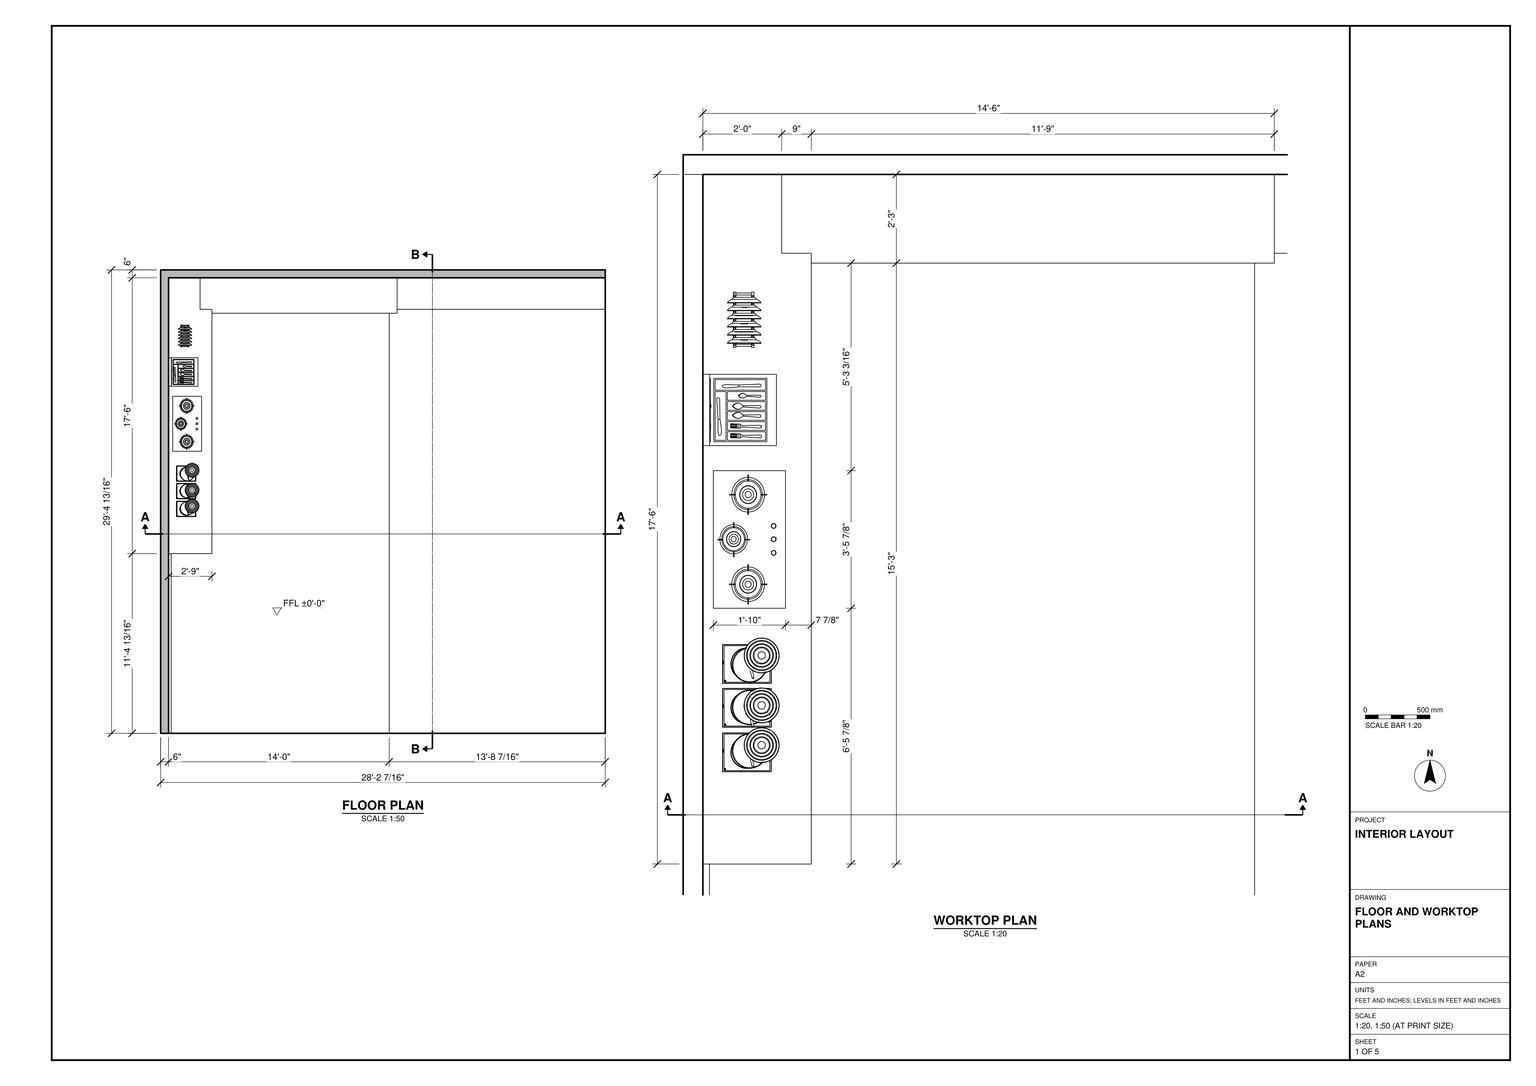
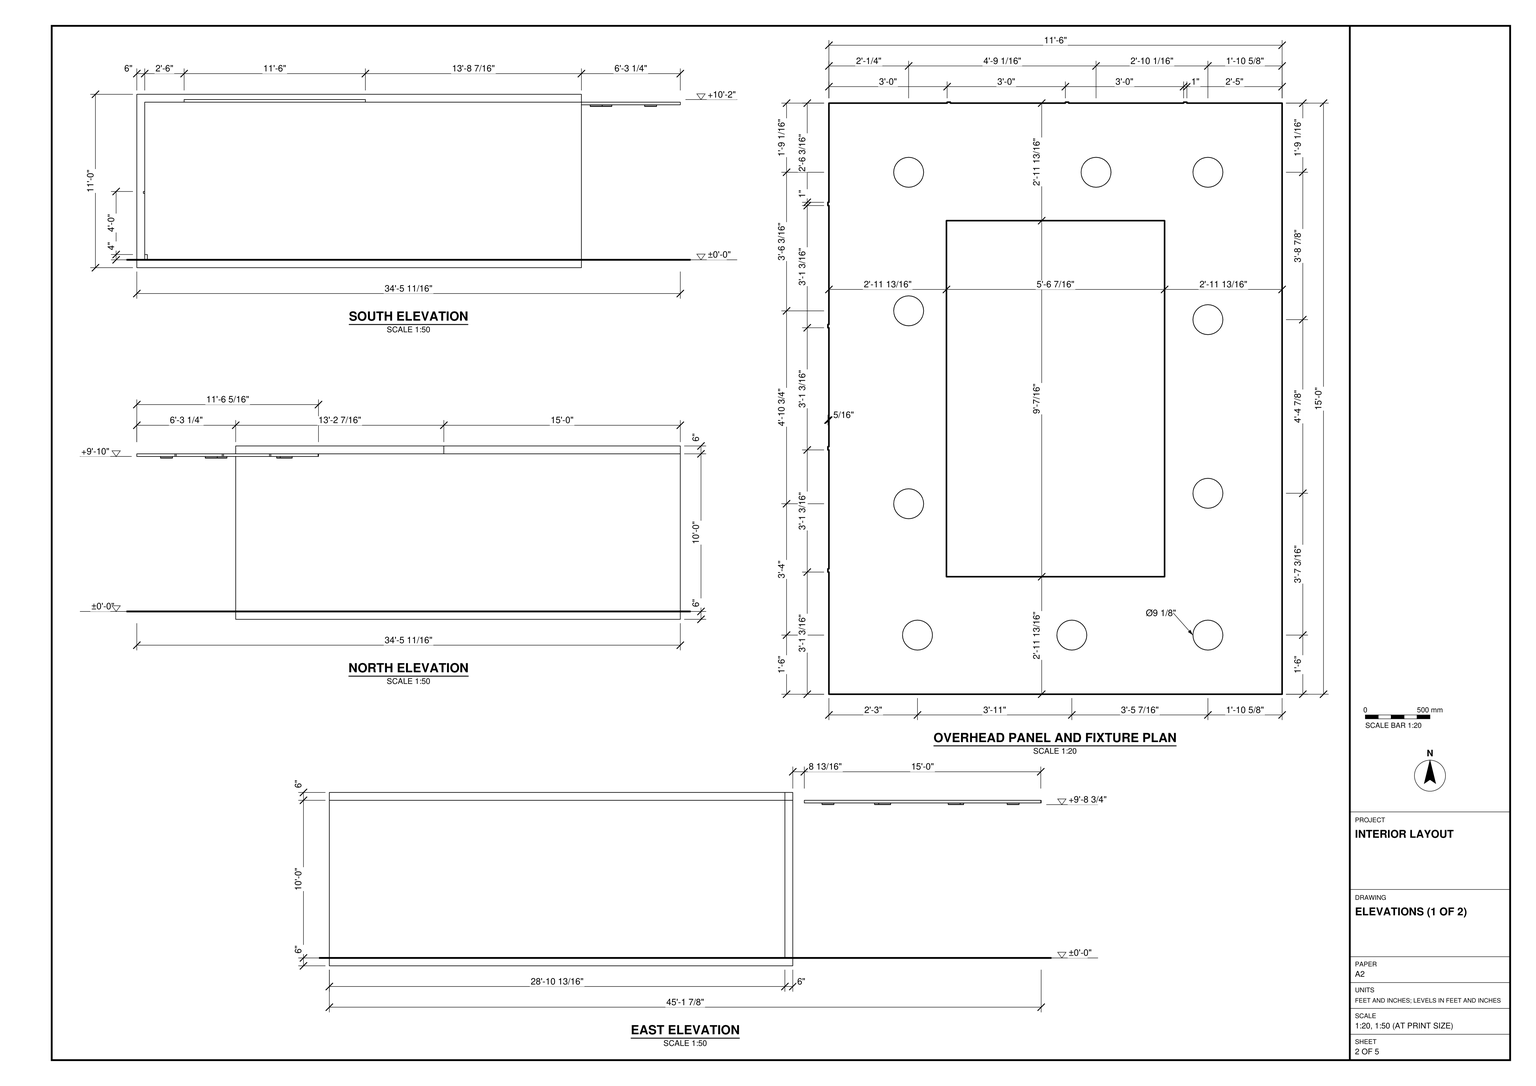
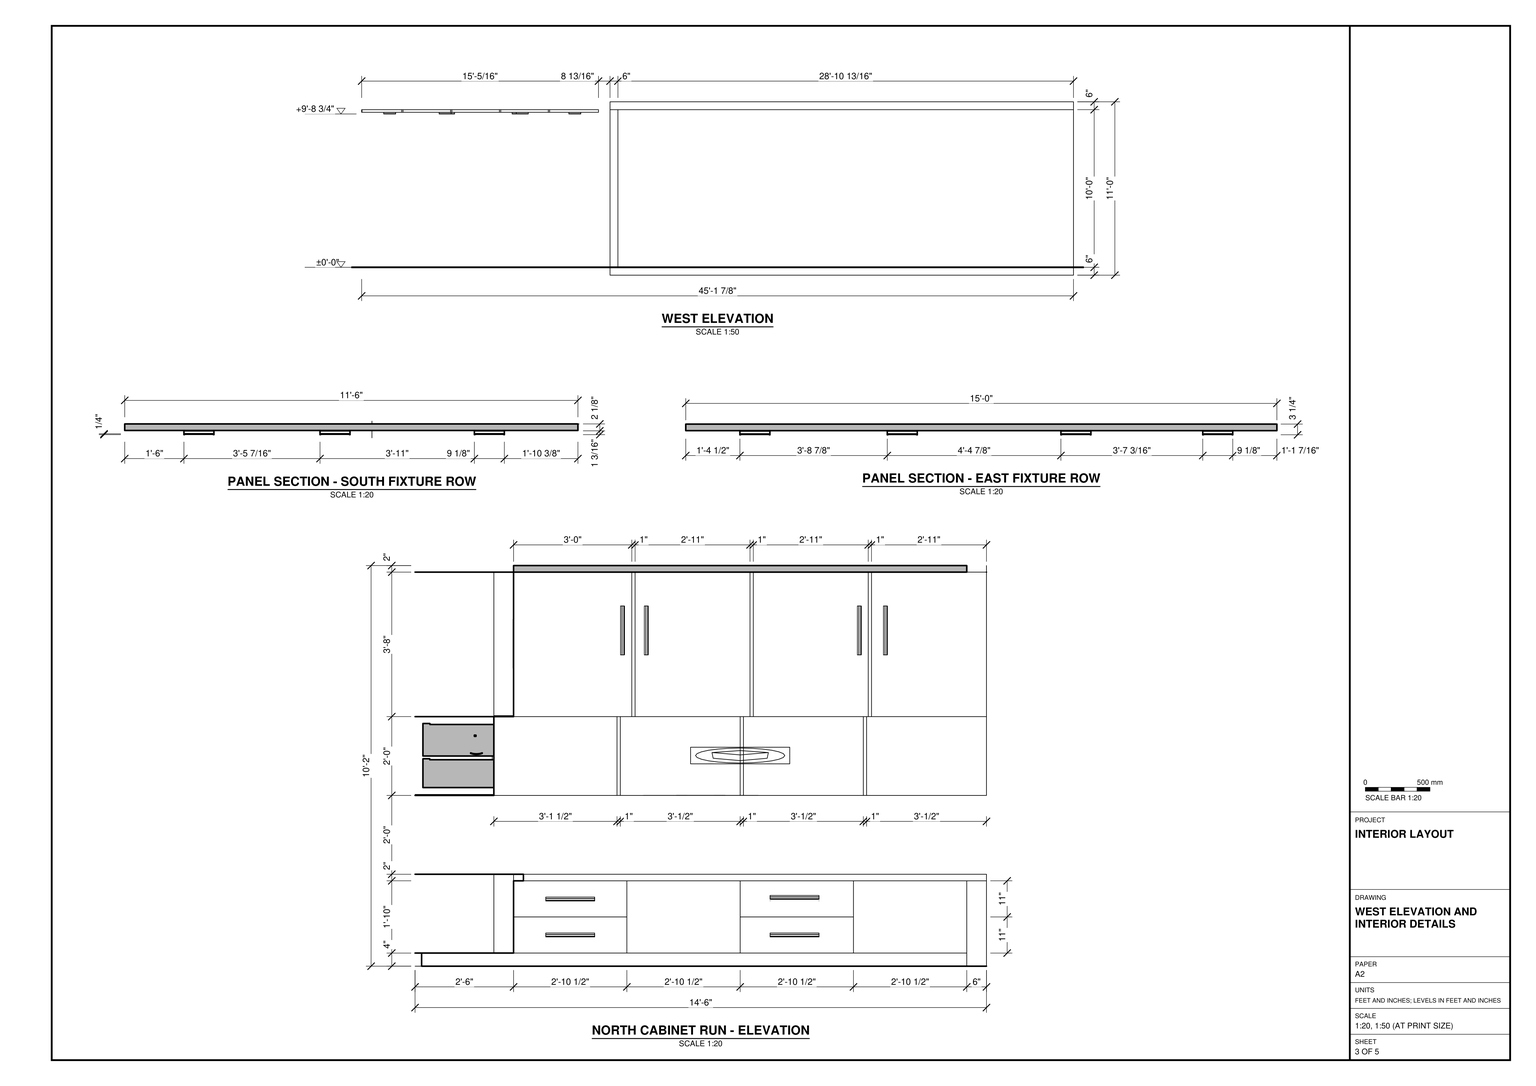
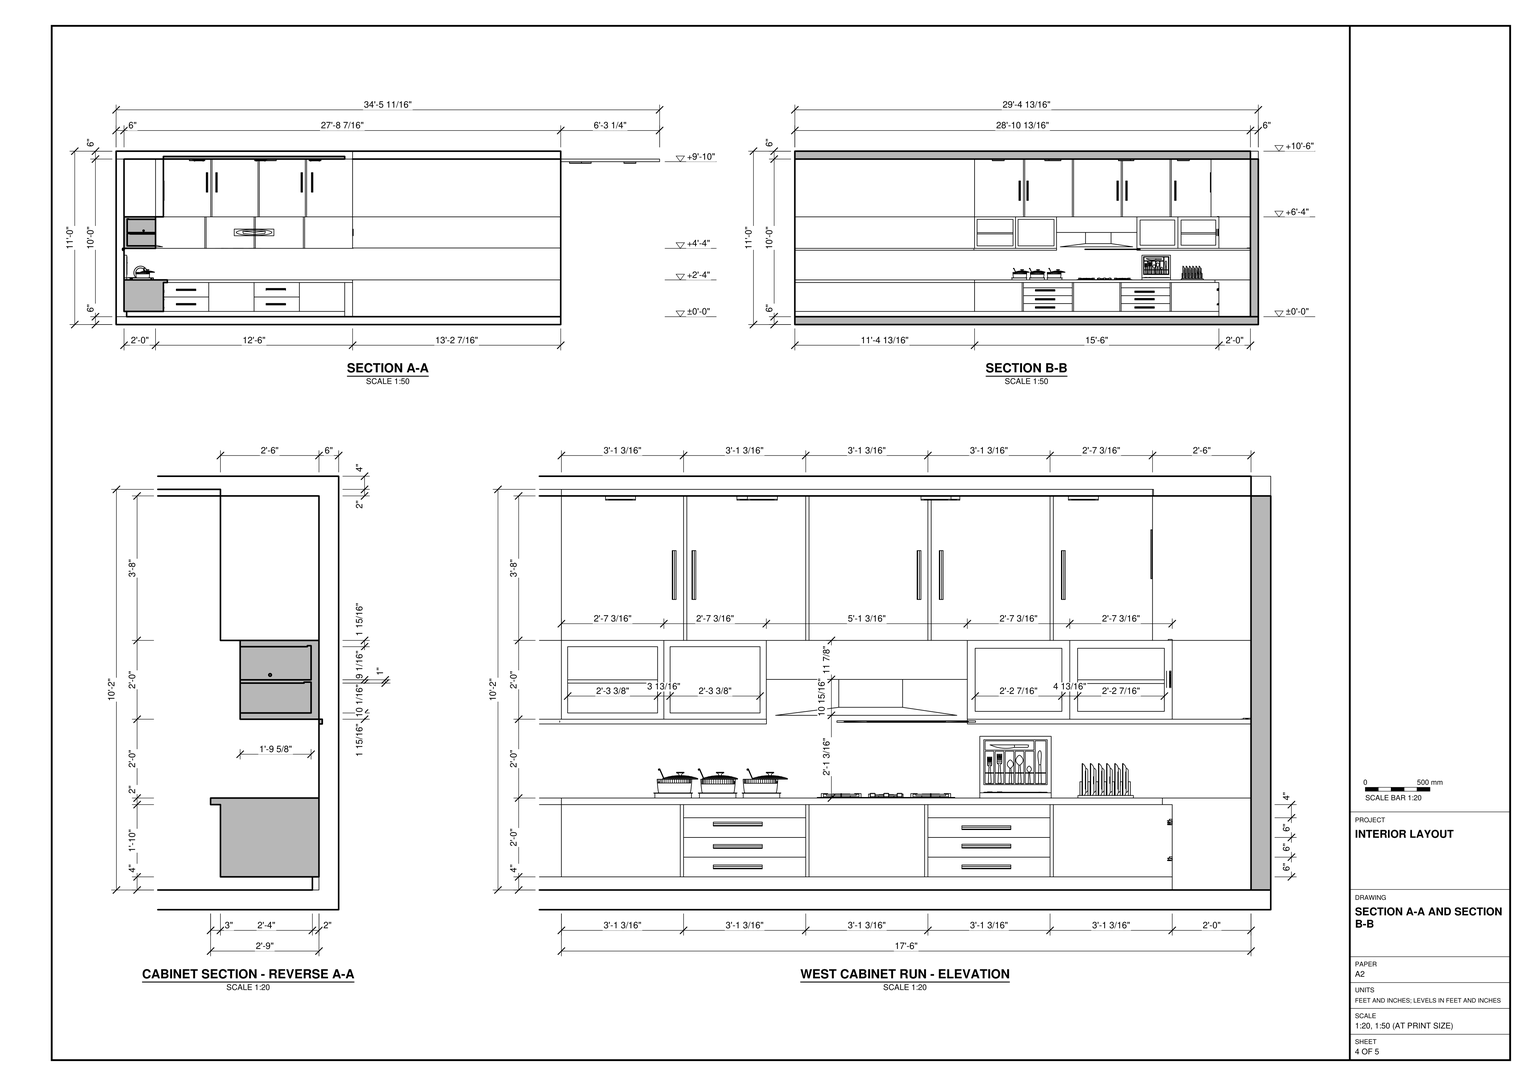
Build the kitchen interior in SketchUp from task_files/diagram_01.pdf. Work in feet and inches. The complete model, including the separate overhead panel, measures 34'-5 11/16" along X, 45'-1 7/8" along Y and 11'-0" along Z. Set the finished floor at ±0'-0". Use the floor plan for the room footprint rather than treating the overall model extents as wall lengths.

Model the floor slab, the adjoining north and west walls, and the slab above the room. Follow the 6" shell thicknesses and the 10'-0" clear height shown in the plans and elevations. Fit the worktop along the west wall and turn it along the north wall, leaving the main floor area open. Match the stepped outline at the corner. Use the north cabinet elevation to set out the plinth, alternating drawer stacks and plain base fronts, the clear space above the worktop, and the two tiers of wall cabinetry. Place the cooktop, utensil tray and cookware in their indicated positions on the west run.

Model the separate overhead panel at the offset shown in the elevations, with its central rectangular field and the fixtures arranged around it. Decor and loose items may be any suitable library components. Keep the shell elements and each furniture or joinery piece in separate groups or components, and use components for repeated parts. Save one SketchUp model as output_files/kitchen_with_l_shaped_joinery_and_overhead_panel.skp.

# SketchUp Ruby script. Lengths in inches.
U = 1.inch
M = Sketchup.active_model
def pt(a) = Geom::Point3d.new(a.map { |v| v * U })
def face(e, loops, mat)
  f = e.add_face(loops[0].map { |a| pt(a) })
  loops[1..].each { |l| e.add_face(l.map { |a| pt(a) }).erase! }
  f.material = f.back_material = mat if mat
  f
end
# faces: each face lists its corners as indices into pts; further lists are holes
def faces(e, pts, list, mat = nil) = list.each { |f| face(e, (f[0].is_a?(Array) ? f : [f]).map { |l| l.map { |i| pts[i] } }, mat) }
# xy, xz, yz: faces in a plane at the given z, y or x. An outline is a flat list of corners, or four numbers for a rectangle; further outlines are holes
def ring(l) = l.size == 4 ? [[l[0], l[1]], [l[2], l[1]], [l[2], l[3]], [l[0], l[3]]] : l.each_slice(2).to_a
def flat(e, list, mat, &to3) = list.each { |f| face(e, (f[0].is_a?(Array) ? f : [f]).map { |l| ring(l).map { |u, v| to3.(u, v) } }, mat) }
def xy(e, z, list, mat = nil) = flat(e, list, mat) { |x, y| [x, y, z] }
def xz(e, y, list, mat = nil) = flat(e, list, mat) { |x, z| [x, y, z] }
def yz(e, x, list, mat = nil) = flat(e, list, mat) { |y, z| [x, y, z] }
def lines(e, pts, list) = list.each { |a, b| e.add_line(pt(pts[a]), pt(pts[b])) }
# prism: a flat outline (further loops are holes) pulled along v
def prism(e, loops, v, mat = nil)
  f = face(e, loops, mat); d = Geom::Vector3d.new(v.map { |x| x * U })
  f.pushpull(f.normal.samedirection?(d) ? d.length : -d.length)
end
def box(e, o, s, mat = nil) = prism(e, [[o, [o[0] + s[0], o[1], o[2]], [o[0] + s[0], o[1] + s[1], o[2]], [o[0], o[1] + s[1], o[2]]]], [0, 0, s[2]], mat)
def at(x, y, z, deg = 0) = Geom::Transformation.translation(pt([x, y, z])) * Geom::Transformation.rotation(ORIGIN, Z_AXIS, deg.degrees)
def axes(o, x, y, z) = Geom::Transformation.new([*x, 0, *y, 0, *z, 0, *pt(o).to_a, 1])
def part(name) = M.definitions.add(name)
# library, detail: a bought-in or finely detailed component or shape, given as its bounding box
def library(name, o, s) = part(name).tap { |d| box(d.entities, o, s) }
def detail(e, o, s) = box(e.add_group.entities, o, s)
def put(e, d, t, mat = nil) = e.add_instance(d, t).tap { |i| i.material = mat if mat }
def group(e, t, mat = nil) = e.add_group.tap { |g| g.transformation = t; g.material = mat if mat }.entities
root = M.entities
M.materials.add("Color_0").color = [255, 255, 255]
M.materials.add("DefaultMaterial32").color = [145, 100, 66]
M.materials.add("Generic").color = [223, 223, 223]
M.materials.add("Teddy_Shoes").color = [231, 232, 232]
M.materials.add("[Carrera Marble]").color = [207, 207, 207]
M.materials.add("[Carrera Marble]2").color = [207, 207, 207]
M.materials.add("[Carrera Marble]3").color = [207, 207, 207]
M.materials.add("[Color_003]").color = [232, 232, 232]
M.materials.add("[Translucent Glass Gray]").color = [128, 128, 128]
M.materials["[Translucent Glass Gray]"].alpha = 0.5
M.materials.add("[_0060_GrassGreen_]").color = [200, 200, 200]
c1 = library("Bosch Stove",[0,0,0],[36.22,20.12,1.38])
c2 = library("PLATE",[-1.81,0,33.86],[10.25,10.83,10.53])
c3 = library("bottle",[0,0,0],[211.8125,112.55,469.29])
c4 = library("top",[0,0,0],[118.11,118.11,64.96])
c5 = library("pump",[0,0,-431.92],[75.04,51.18,479.16])
c6 = library("cap",[0,0,0],[90.55,90.55,133.86])
c7 = library("Group\#3",[0,0,0],[19.58,60.1,12.07])
c8 = part("E")
xy(c8.entities,0.2,[[6.05,0,4.93,0.4,4.54,0.95,4.41,1.79,4.41,31.375,4.54,32.22,4.93,32.77,6.05,33.17,21.79,33.17,22.16,33.06,22.43,32.73,22.59,32.15,22.66,31.3,22.59,30.49,22.43,29.92,22.16,29.6,21.79,29.5,8.82,29.5,8.82,19.1,19.94,19.1,20.3125,18.98,20.59,18.66,20.76,18.1,20.8125,17.25,20.76,16.46,20.59,15.92,20.3125,15.62,19.94,15.53,8.82,15.53,8.82,3.67,21.97,3.67,22.34,3.5625,22.63,3.24,22.8125,2.68,22.86,1.82,22.8125,1.01,22.63,0.4375,22.34,0.1,21.97,0]])
c9 = part("S")
xy(c9.entities,0.2,[[10.94,0,7.86,0.28,5.32,0.97,3.45,1.82,2.4,2.5625,1.96,3.34,1.82,4.61,1.87,5.55,2.02,6.15,2.28,6.47,2.64,6.5625,3.65,6.125,5.33,5.18,7.8,4.22,11.15,3.77,13.78,4.15,15.83,5.24,17.15,6.97,17.61,9.3,17.45,10.61,16.97,11.71,15.28,13.47,12.88,14.85,10.125,16.14,7.38,17.58,5,19.45,3.29,21.98,2.8,23.57,2.64,25.45,2.83,27.42,3.4,29.16,4.3,30.65,5.5,31.89,6.97,32.86,8.7,33.56,10.63,34,12.71,34.14,14.93,33.95,17.03,33.4375,18.79,32.72,19.8,32.08,20.12,31.69,20.25,31.33,20.33,30.81,20.35,30.01,20.3125,29.19,20.2,28.59,19.98,28.23,19.66,28.12,18.78,28.48,17.3,29.28,15.24,30.1,12.56,30.48,10.15,30.1,8.46,29.12,7.46,27.66,7.125,25.86,7.29,24.57,7.77,23.48,9.47,21.71,11.89,20.3,14.66,19.01,17.43,17.57,19.85,15.72,21.57,13.21,22.06,11.63,22.22,9.79,22.01,7.59,21.36,5.64,20.34,3.96,18.98,2.55,17.32,1.4375,15.39,0.64,13.25,0.16]])
c10 = part("S\#2")
xy(c10.entities,0.08,[[4.38,0,3.14,0.11,2.13,0.39,1.38,0.73,0.96,1.03,0.78,1.34,0.73,1.85,0.75,2.22,0.81,2.46,0.91,2.59,1.06,2.625,1.46,2.45,2.13,2.07,3.12,1.6875,4.46,1.51,5.51,1.66,6.33,2.1,6.86,2.79,7.04,3.72,6.98,4.24,6.79,4.69,6.11,5.39,5.15,5.94,4.05,6.45,2.95,7.03,2,7.78,1.32,8.79,1.12,9.43,1.06,10.18,1.13,10.97,1.36,11.66,1.72,12.26,2.2,12.75,2.79,13.14,3.48,13.43,4.25,13.6,5.09,13.66,5.97,13.58,6.8125,13.375,7.52,13.09,7.92,12.83,8.05,12.68,8.1,12.53,8.13,12.32,8.14,12.01,8.125,11.68,8.08,11.4375,7.99,11.29,7.86,11.25,7.51,11.39,6.92,11.71,6.1,12.04,5.02,12.19,4.06,12.04,3.38,11.65,2.98,11.0625,2.85,10.34,2.91,9.83,3.11,9.39,3.79,8.68,4.76,8.12,5.86,7.6,6.97,7.03,7.94,6.29,8.63,5.29,8.82,4.65,8.89,3.92,8.8,3.03,8.55,2.26,8.14,1.58,7.59,1.02,6.93,0.58,6.16,0.26,5.3,0.0625]])
c11 = part("E\#2")
xy(c11.entities,0.08,[[2.42,0,1.97,0.16,1.82,0.38,1.76,0.72,1.76,12.55,1.82,12.89,1.97,13.11,2.42,13.27,8.71,13.27,8.86,13.23,8.97,13.09,9.04,12.86,9.0625,12.52,9.04,12.2,8.97,11.97,8.86,11.84,8.71,11.8,3.53,11.8,3.53,7.64,7.98,7.64,8.125,7.59,8.24,7.46,8.3,7.24,8.33,6.9,8.3,6.58,8.24,6.37,8.125,6.25,7.98,6.21,3.53,6.21,3.53,1.47,8.79,1.47,8.94,1.43,9.05,1.3,9.125,1.07,9.15,0.73,9.125,0.4,9.05,0.17,8.94,0.04,8.79,0]])
c12 = part("C")
xy(c12.entities,0.2,[[16.56,0,13.49,0.27,10.73,1.08,8.32,2.41,6.29,4.25,4.67,6.6,3.47,9.45,2.73,12.77,2.49,16.56,2.75,20.46,3.55,23.91,4.83,26.9,6.54,29.39,8.65,31.36,11.14,32.81,13.96,33.69,17.07,33.99,19.86,33.72,22.375,33.04,24.43,32.09,25.67,31.21,26.12,30.68,26.29,30.26,26.39,29.68,26.43,28.89,26.375,28.02,26.22,27.41,25.98,27.05,25.63,26.9375,24.63,27.4375,22.98,28.54,20.52,29.64,17.04,30.14,14.94,29.92,13.03,29.26,11.36,28.17,9.95,26.66,8.81,24.75,7.96,22.47,7.43,19.82,7.25,16.8125,7.42,13.84,7.93,11.24,8.76,9.02,9.88,7.19,11.29,5.76,13,4.73,14.96,4.1,17.17,3.9,20.62,4.38,23.13,5.47,24.84,6.5625,25.89,7.05,26.2,6.97,26.4,6.68,26.52,6.07,26.55,5.1,26.53,4.38,26.4375,3.84,26.27,3.43,25.91,3,24.84,2.22,22.8,1.19,20.01,0.35]])
c13 = part("L")
xy(c13.entities,0.08,[[2.42,0,1.97,0.16,1.82,0.38,1.76,0.72,1.76,13,1.8,13.14,1.95,13.24,2.22,13.3,2.65,13.33,3.07,13.3,3.34,13.24,3.49,13.14,3.53,13,3.53,1.53,8.28,1.53,8.44,1.48,8.56,1.35,8.62,1.12,8.64,0.77,8.62,0.43,8.56,0.19,8.44,0.05,8.28,0]])
c14 = part("M\#1")
xy(c14.entities,0.08,[[2.6,0,2.19,0.03,1.93,0.09,1.8,0.18,1.76,0.33,1.76,12.53,1.82,12.9,1.99,13.14,2.49,13.33,3.56,13.33,4.13,13.27,4.5625,13.07,4.87,12.73,5.09,12.25,8.93,2.65,8.98,2.65,12.98,12.22,13.23,12.74,13.52,13.09,13.87,13.27,14.32,13.33,15.44,13.33,15.73,13.28,15.97,13.14,16.13,12.89,16.1875,12.53,16.1875,0.33,16.15,0.18,16,0.09,15.74,0.03,15.33,0,14.92,0.03,14.66,0.09,14.52,0.18,14.48,0.33,14.48,11.88,14.46,11.88,9.73,0.28,9.64,0.15,9.48,0.07,9.22,0.02,8.87,0,8.5,0.02,8.24,0.08,8.08,0.16,8.01,0.28,3.49,11.88,3.48,11.88,3.48,0.33,3.43,0.18,3.29,0.09,3.02,0.03]])
c15 = part("A\#2")
xy(c15.entities,0.2,[[[2.97,0,1.76,0.0625,1.09,0.31,0.91,0.83,1.13,1.74,12.25,32.55,12.52,33.01,13.01,33.3,13.83,33.4375,15.1,33.47,16.46,33.4375,17.33,33.3,17.84,33,18.12,32.53,29.25,1.72,29.46,0.81,29.27,0.28,28.59,0.05,27.32,0,26.05,0.04,25.34,0.17,24.98,0.41,24.76,0.79,21.91,8.87,8.125,8.87,5.41,0.9,5.2,0.5,4.83,0.22,4.14,0.05],[9.23,12.38,20.76,12.38,14.97,28.91,14.94,28.91]]])
c16 = part("K")
xy(c16.entities,0.08,[[2.65,0,2.22,0.03,1.95,0.09,1.8,0.19,1.76,0.33,1.76,13.0625,1.8,13.21,1.95,13.3,2.22,13.36,2.65,13.39,3.07,13.36,3.34,13.3,3.49,13.21,3.53,13.0625,3.53,7.17,8.22,13.0625,8.37,13.22,8.57,13.3125,8.85,13.37,9.29,13.39,9.72,13.36,9.98,13.3,10.11,13.2,10.15,13.0625,10.08,12.8,9.83,12.43,5.43,7.17,10.17,0.87,10.38,0.51,10.42,0.35,10.38,0.2,10.24,0.09,9.97,0.03,9.51,0,8.93,0.03,8.59,0.14,8.41,0.33,3.53,6.96,3.53,0.33,3.49,0.19,3.34,0.09,3.07,0.03]])
c17 = part("A\#3")
xy(c17.entities,0.2,[[[2.97,0,1.76,0.0625,1.09,0.31,0.91,0.83,1.13,1.74,12.25,32.55,12.52,33.01,13.01,33.3,13.83,33.4375,15.1,33.47,16.46,33.4375,17.33,33.3,17.84,33,18.12,32.53,29.25,1.72,29.46,0.81,29.27,0.28,28.59,0.05,27.32,0,26.05,0.04,25.34,0.17,24.98,0.41,24.76,0.79,21.91,8.87,8.125,8.87,5.41,0.9,5.2,0.5,4.83,0.22,4.14,0.05],[9.23,12.38,20.76,12.38,14.97,28.91,14.94,28.91]]])
c18 = part("D")
xy(c18.entities,0.2,[[[6.05,0,4.93,0.4,4.54,0.95,4.41,1.79,4.41,31.375,4.54,32.22,4.93,32.77,6.05,33.17,13.56,33.17,17.53,32.89,20.84,32.05,23.57,30.69,25.82,28.85,27.59,26.54,28.875,23.79,29.65,20.62,29.91,17.07,29.64,13.04,28.81,9.55,27.45,6.61,25.59,4.22,23.24,2.37,20.4,1.05,17.03,0.26,13.07,0],[8.82,3.69,13.35,3.69,16.28,3.89,18.71,4.49,20.71,5.49,22.35,6.92,23.63,8.77,24.54,11.03,25.09,13.74,25.27,16.89,25.11,19.49,24.61,21.9,23.75,24.06,22.52,25.91,20.91,27.42,18.92,28.55,16.42,29.26,13.3,29.5,8.82,29.5]]])
c19 = part("O\#1")
xy(c19.entities,0.08,[[[6.82,0,5.42,0.11,4.23,0.45,3.23,0.99,2.42,1.74,1.8,2.7,1.36,3.85,1.1,5.21,1.02,6.76,1.11,8.25,1.39,9.61,1.87,10.79,2.53,11.79,3.39,12.58,4.43,13.17,5.66,13.53,7.08,13.66,8.46,13.55,9.64,13.22,10.63,12.67,11.45,11.93,12.08,10.98,12.52,9.84,12.79,8.5,12.88,6.98,12.78,5.45,12.5,4.08,12.03,2.88,11.37,1.88,10.52,1.08,9.47,0.49,8.24,0.12],[6.91,1.53,7.98,1.64,8.86,1.96,9.57,2.46,10.13,3.12,10.54,3.91,10.82,4.82,11.02,6.86,10.82,8.96,10.56,9.86,10.16,10.64,9.61,11.27,8.91,11.75,8.04,12.05,6.98,12.15,5.93,12.04,5.05,11.72,4.35,11.22,3.79,10.57,3.37,9.79,3.09,8.89,2.88,6.88,3.08,4.73,3.34,3.81,3.73,3.03,4.27,2.4,4.97,1.92,5.84,1.625]]])
c20 = part("P")
xy(c20.entities,0.08,[[[2.65,0,2.22,0.03,1.95,0.09,1.8,0.18,1.76,0.33,1.76,12.57,1.82,12.92,1.98,13.15,2.46,13.33,5.3,13.33,6.125,13.29,7.06,13.14,8.16,12.7,9.1,11.9,9.7,10.8125,9.91,9.44,9.83,8.5,9.59,7.65,9.1875,6.91,8.65,6.28,7.97,5.79,7.15,5.41,6.18,5.18,5.03,5.11,3.53,5.11,3.53,0.33,3.48,0.18,3.34,0.09,3.07,0.03],[3.53,6.55,5.12,6.55,5.85,6.6,6.44,6.76,7.33,7.33,7.875,8.2,8.06,9.3,7.98,10.04,7.76,10.65,7.42,11.125,7.01,11.46,6.08,11.8,5.16,11.87,3.53,11.87]]])
c21 = part("O")
xy(c21.entities,0.08,[[[6.82,0,5.42,0.11,4.23,0.45,3.23,0.99,2.42,1.74,1.8,2.7,1.36,3.85,1.1,5.21,1.02,6.76,1.11,8.25,1.39,9.61,1.87,10.79,2.53,11.79,3.39,12.58,4.43,13.17,5.66,13.53,7.08,13.66,8.46,13.55,9.64,13.22,10.63,12.67,11.45,11.93,12.08,10.98,12.52,9.84,12.79,8.5,12.88,6.98,12.78,5.45,12.5,4.08,12.03,2.88,11.37,1.88,10.52,1.08,9.47,0.49,8.24,0.12],[6.91,1.53,7.98,1.64,8.86,1.96,9.57,2.46,10.13,3.12,10.54,3.91,10.82,4.82,11.02,6.86,10.82,8.96,10.56,9.86,10.16,10.64,9.61,11.27,8.91,11.75,8.04,12.05,6.98,12.15,5.93,12.04,5.05,11.72,4.35,11.22,3.79,10.57,3.37,9.79,3.09,8.89,2.88,6.88,3.08,4.73,3.34,3.81,3.73,3.03,4.27,2.4,4.97,1.92,5.84,1.625]]])
c22 = part("N")
xy(c22.entities,0.08,[[2.59,0,2.1875,0.03,1.9375,0.09,1.8,0.19,1.76,0.33,1.76,12.57,1.82,12.92,1.99,13.15,2.48,13.33,3.32,13.33,3.82,13.28,4.18,13.11,4.49,12.78,4.81,12.25,8.03,6.43,8.6,5.39,9.14,4.39,9.64,3.42,10.14,2.46,10.15,2.46,10.125,4.15,10.12,5.83,10.12,13.03,10.16,13.16,10.3,13.27,10.56,13.34,10.97,13.36,11.36,13.34,11.62,13.27,11.75,13.16,11.79,13.03,11.79,0.79,11.72,0.44,11.55,0.21,11.31,0.07,11.04,0.03,10.48,0.03,10.01,0.09,9.63,0.29,9.27,0.7,8.88,1.35,4.7,8.9,4.03,10.125,3.41,11.37,3.39,11.37,3.42,9.86,3.43,8.34,3.43,0.33,3.39,0.19,3.26,0.09,3,0.03]])
c23 = part("R")
xy(c23.entities,0.08,[[[2.65,0,2.22,0.03,1.95,0.09,1.8,0.18,1.76,0.33,1.76,12.61,1.82,12.95,1.97,13.17,2.42,13.33,5.24,13.33,6.07,13.3,6.67,13.25,8.03,12.83,8.58,12.5,9.02,12.1,9.37,11.625,9.62,11.09,9.82,9.83,9.64,8.64,9.125,7.7,8.31,7,7.26,6.5,7.85,6.14,8.35,5.61,8.79,4.9,9.2,4,10.39,1.08,10.57,0.56,10.61,0.33,10.58,0.18,10.45,0.08,10.16,0.02,9.67,0,9.23,0.02,8.96,0.09,8.8,0.22,8.7,0.42,7.48,3.55,7.04,4.53,6.49,5.3,5.74,5.8,4.71,5.98,3.53,5.98,3.53,0.33,3.48,0.18,3.34,0.09,3.07,0.03],[3.53,7.4,5.25,7.4,6.45,7.57,7.3,8.04,7.8,8.76,7.96,9.65,7.87,10.37,7.61,10.97,7.14,11.43,6.4375,11.74,5.86,11.84,5.01,11.87,3.53,11.87]]])
c24 = part("A\#4")
xy(c24.entities,0.08,[[[1.1875,0,0.7,0.03,0.4375,0.125,0.36,0.33,0.45,0.7,4.9,13.02,5.01,13.21,5.2,13.32,5.53,13.375,6.04,13.39,6.58,13.375,6.93,13.32,7.14,13.2,7.25,13.01,11.7,0.6875,11.79,0.32,11.71,0.11,11.4375,0.02,10.93,0,10.42,0.02,10.13,0.07,9.99,0.16,9.9,0.32,8.77,3.55,3.25,3.55,2.16,0.36,2.08,0.2,1.93,0.09,1.66,0.02],[3.69,4.95,8.3,4.95,5.99,11.56,5.98,11.56]]])
c25 = part("moon+sparkle1")
put(c25.entities,c3,at(-105.91,-56.27,0))
put(c25.entities,c4,at(-59.06,-59.06,420.08))
put(c25.entities,c5,at(-25.59,-25.59,465.35))
put(c25.entities,c6,at(-45.28,-45.28,465.35))
put(c25.entities,c7,at(-26.48,37.05,446.59,-180))
put(c25.entities,c7,at(26.48,-37.05,446.59))
g1 = group(c25.entities,at(-71.56,-56.01,283.65))
put(g1,c8,axes([-3.4,19.97,29.22],[0.8143,-0.38329,0],[-0.00323,-0.00686,0.89997],[-0.42586,-0.90475,-0.00842]))
put(g1,c9,axes([21.14,9.23,28.7],[0.85645,-0.27657,0],[-0.0032,-0.00991,0.89994],[-0.30728,-0.95155,-0.01157]))
put(g1,c10,axes([62.22,1.25,0],[0.99807,-0.06205,0],[-0.00072,-0.01159,0.99993],[-0.06204,-0.99801,-0.01161]))
put(g1,c11,axes([135.94,15.27,0.32],[0.9059,0.42349,0],[0.0031,-0.00664,0.99997],[0.42348,-0.90588,-0.00733]))
put(g1,c12,axes([44.22,2.03,29.27],[0.89822,-0.05653,0],[-0.00071,-0.01134,0.89993],[-0.0628,-0.99795,-0.01263]))
put(g1,c13,axes([124.12,10.23,0.5],[0.95161,0.3073,0],[0.00284,-0.00878,0.99996],[0.30728,-0.95157,-0.00923]))
put(g1,c14,axes([-1.27,19.22,0.39],[0.9059,-0.42349,0],[-0.0031,-0.00664,0.99997],[-0.42348,-0.90588,-0.00733]))
put(g1,c15,axes([74.38,0.48,29.71],[0.80842,0.05057,0],[0.00072,-0.01156,0.89993],[0.06242,-0.99797,-0.01286]))
put(g1,c16,axes([112.06,6.35,0.16],[0.9522,0.30547,0],[0.00319,-0.00994,0.99995],[0.30545,-0.95215,-0.01044]))
put(g1,c17,axes([130.05,12.23,30.39],[0.73378,0.34303,0],[0.00385,-0.00823,0.89995],[0.42347,-0.90586,-0.01009]))
put(g1,c18,axes([99.8125,2.06,29.73],[0.85645,0.27657,0],[0.0032,-0.00991,0.89994],[0.30728,-0.95155,-0.01157]))
put(g1,c19,axes([29.59,6.23,0.29],[0.98249,-0.18632,0],[-0.00197,-0.0104,0.99994],[-0.18631,-0.98243,-0.01058]))
put(g1,c20,axes([73.19,0.77,0.02],[0.99807,0.06205,0],[0.00072,-0.01159,0.99993],[0.06204,-0.99801,-0.01161]))
put(g1,c21,axes([15.85,11.25,0.32],[0.95161,-0.3073,0],[-0.00284,-0.00878,0.99996],[-0.30728,-0.95157,-0.00923]))
put(g1,c22,axes([43.47,3.6,0.32],[0.9827,-0.18518,0],[-0.00209,-0.01111,0.99994],[-0.18517,-0.98264,-0.01131]))
put(g1,c23,axes([99.65,3.6,0.32],[0.9827,0.18518,0],[0.00209,-0.01111,0.99994],[0.18517,-0.98264,-0.01131]))
put(g1,c24,axes([85.625,1.53,0.78],[0.99805,0.06243,0],[0.00071,-0.01135,0.99994],[0.06243,-0.99798,-0.01137]))
c26 = library("Cutlery organizer",[0,0,0],[15.54,15.48,15.54])
c27 = library("스마트바손잡이",[-0.08,-0.03,8.9],[0.83,23.68,1.89])
c28 = library("1007",[-3.54,-4.03,0],[7.08,8.26,3.15])
c29 = library("bowl",[0,0.89,0],[17.28,40.76,9.89])
c30 = library("Plate rack",[-0.65,-0.94,-0.7],[10.38,9.93,9.93])
c31 = library("VintageView+Vino+-+Pins",[378.17,33.06,-0.08],[10.85,4.5,3.85])
c32 = library("Spoon+stand",[-0.92,0,0],[11.25,4.72,10.63])
c33 = library("Tlon Light 650 Ceiling 152 007",[-12.8,-12.8,-3.78],[25.6,25.6,3.58])
c34 = library("Mesh Light",[-0.5,-0.5,-0.1],[1,1,0.2])
c35 = library("Group\#4",[-0.5,-0.5,0],[3.13,182.7,11.22])
c36 = library("Group\#14",[-0.5,-0.5,0],[175,3.47,0.3])
c37 = library("Group\#15",[-0.5,-0.5,0],[151,2.22,24.3])
xy(root,-6,[[0,0,338.4375,352.8125]])
xy(root,0,[[174,322.8125,180,346.8125],[180,322.8125,338.4375,346.8125],[8,344.8125,8,346.8125,0,346.8125,0,352.8125,338.4375,352.8125,338.4375,346.8125,174,346.8125,174,344.8125]])
xy(root,0,[[8,0,174,344.8125],[174,0,338.4375,322.8125]],"Generic")
xy(root,4,[[6,0,8,136.8125],[6,136.8125,8,346.8125],[8,136.8125,8,344.8125,30,344.8125,30,322.8125,36,322.8125,36,286.61,35.7,286.61,35.7,285.61,36,285.61,36,248.41,35.7,248.41,35.7,247.41,36,247.41,36,212.21,35.7,212.21,35.7,211.21,36,211.21,36,174.01,35.7,174.01,35.7,173.01,36,173.01,36,136.8125],[30,322.8125,174,344.8125],[8,344.8125,30,346.8125],
  [30,344.8125,174,346.8125]])
xy(root,26,[[36,136.8125,39,173.01],[35.7,173.01,36,174.01],[36,173.01,39,174.01],[35.7,174.01,36,211.21],[36,174.01,39,211.21],
  [35.7,211.21,36,212.21],[36,211.21,39,212.21],[36,212.21,39,247.41],[35.7,247.41,36,248.41],[36,247.41,39,248.41],
  [36,248.41,39,285.61],[35.7,285.61,39,286.61],[36,286.61,39,322.8125],[39,319.8125,70.5,322.8125],[70.5,319.8125,105,322.8125],
  [105,319.8125,139.5,322.8125],[139.5,319.8125,174,322.8125],[174,319.8125,180,322.8125]])
xy(root,28,[[6,136.8125,39,136.8125,39,322.8125,30,322.8125,30,346.8125,6,346.8125],[39,319.8125,180,319.8125,180,346.8125,30,346.8125,30,322.8125,39,322.8125]],"[Carrera Marble]3")
xy(root,50.5625,[[5,0,5.5,136.8125],[5.5,0,6,136.8125]])
xy(root,52,[[5,0,6,199.21],[6,136.8125,30,199.21],[5,199.21,6,199.25],[5,260.41,6,346.8125],[6,260.41,30,344.35],
  [30,322.8125,30,344.35,180,344.35,180,322.8125,143.5,322.8125,143.5,323.11,142.5,323.11,142.5,322.8125,106,322.8125,106,323.11,105,323.11,105,322.8125,68.5,322.8125,68.5,323.11,67.5,323.11,67.5,322.8125]])
xy(root,53.1875,[[12.95,202.03,35.39,257.25]])
xy(root,53.91,[[8.4,138.72,30,166.1],[8.4,169.92,30,197.3]])
xy(root,54.39,[[8.4,262.8,30,289.22],[8.4,294,30,320.42]])
xy(root,55.625,[[12.95,221.28,24.7,240.72]])
xy(root,62.875,[[10.48,294,30,320.42]])
xy(root,63,[[10.53,138.72,30,166.1]])
xy(root,64,[[8.4,138.72,30,166.1],[8.4,294,30,320.42]])
xy(root,64.125,[[[6,199.21,30,260.41],[12.95,221.28,24.7,240.72]]])
xy(root,73.61,[[10.53,262.8,30,272.14],[10.53,272.14,30,285.61],[10.53,285.61,30,289.22],[10.53,294,30,320.42]])
xy(root,74.09,[[9.55,138.72,30,166.1],[10.53,169.92,30,174.01],[10.53,174.01,30,197.3]])
xy(root,74.39,[[8.4,169.92,10.53,174.01]])
xy(root,76,[[6,136.8125,30,346.8125],[30,136.8125,36,174.01],[30,174.01,30,211.21,36,211.21,36,175.01,35.7,175.01,35.7,174.01],[30,211.21,30,248.41,36,248.41,36,212.21,35.7,212.21,35.7,211.21],[30,248.41,30,272.14,36,272.14,36,249.41,35.7,249.41,35.7,248.41],
  [30,272.14,36,285.61],[30,285.61,30,321.59,36,321.59,36,286.61,35.7,286.61,35.7,285.61],[36,316.8125,67.5,321.59],[67.5,316.8125,68.5,321.59],[68.5,316.8125,72,321.59],
  [73,316.8125,105,321.59],[105,316.8125,106,321.59],[106,316.8125,108,321.59],[109,316.8125,142.5,321.59],[142.5,316.8125,143.5,321.59],
  [143.5,316.8125,144,321.59],[145,316.8125,174,321.59],[174,316.8125,180,321.59],[72,317.11,73,321.59],[108,317.11,109,321.59],
  [144,317.11,145,321.59],[30,322.8125,67.5,322.8125,67.5,323.11,68.5,323.11,68.5,322.8125,105,322.8125,105,323.11,106,323.11,106,322.8125,142.5,322.8125,142.5,323.11,143.5,323.11,143.5,322.8125,174,322.8125,174,346.8125,30,346.8125],[67.5,322.8125,68.5,323.11],[105,322.8125,106,323.11],[142.5,322.8125,143.5,323.11],
  [174,322.8125,180,346.8125]])
xy(root,76.3,[[143.5,321.59,144,322.8125]])
xy(root,76.3,[[142.5,321.59,143.5,322.8125],[144,321.59,145,322.8125]],"Color_0")
xy(root,118,[[[275.72,361.6,275.72,398.8,275.42,398.8,275.42,399.8,275.72,399.8,275.72,436,275.42,436,275.42,437,275.72,437,275.72,473.2,275.42,473.2,275.42,474.2,275.72,474.2,275.72,510.4,275.42,510.4,275.42,511.4,275.72,511.4,275.72,541.6,311.72,541.6,311.72,541.9,312.72,541.9,312.72,541.6,347.72,541.6,347.72,541.9,348.72,541.9,348.72,541.6,383.72,541.6,383.72,541.9,384.72,541.9,384.72,541.6,413.72,541.6,413.72,361.6],[311.51,397.39,377.93,505.8125]]],"[Color_003]")
xy(root,120,[[6,0,36,136.8125],[36,0,174,136.8125],[174,0,338.4375,136.8125],[6,136.8125,6,346.8125,30,346.8125,30,322.8125,36,322.8125,36,286.61,35.7,286.61,35.7,285.61,36,285.61,36,249.41,35.7,249.41,35.7,248.41,36,248.41,36,212.21,35.7,212.21,35.7,211.21,36,211.21,36,175.01,35.7,175.01,35.7,174.01,36,174.01,36,136.8125],[180,136.8125,338.4375,316.8125],
  [36,316.8125,36,322.8125,30,322.8125,30,346.8125,174,346.8125,174,316.8125,145,316.8125,145,317.11,144,317.11,144,316.8125,109,316.8125,109,317.11,108,317.11,108,316.8125,73,316.8125,73,317.11,72,317.11,72,316.8125],[174,316.8125,180,346.8125],[180,316.8125,338.4375,322.8125],[180,322.8125,338.4375,346.8125],[0,346.8125,180,352.8125],
  [180,346.8125,338.4375,352.8125],[[275.72,361.6,413.72,361.6,413.72,541.6,384.72,541.6,384.72,541.9,383.72,541.9,383.72,541.6,348.72,541.6,348.72,541.9,347.72,541.9,347.72,541.6,312.72,541.6,312.72,541.9,311.72,541.9,311.72,541.6,275.72,541.6,275.72,511.4,275.42,511.4,275.42,510.4,275.72,510.4,275.72,474.2,275.42,474.2,275.42,473.2,275.72,473.2,275.72,437,275.42,437,275.42,436,275.72,436,275.72,399.8,275.42,399.8,275.42,398.8,275.72,398.8],[311.51,397.39,377.93,505.8125]],[311.51,397.39,377.93,505.8125]])
xy(root,120,[[[36,136.8125,36,174.01,35.7,174.01,35.7,175.01,36,175.01,36,211.21,35.7,211.21,35.7,212.21,36,212.21,36,248.41,35.7,248.41,35.7,249.41,36,249.41,36,285.61,35.7,285.61,35.7,286.61,36,286.61,36,316.8125,72,316.8125,72,317.11,73,317.11,73,316.8125,108,316.8125,108,317.11,109,317.11,109,316.8125,144,316.8125,144,317.11,145,317.11,145,316.8125,174,316.8125,174,136.8125],[71.79,172.6,138.21,281.03]]],"[Color_003]")
xy(root,122,[[36,0,174,136.8125],[[36,136.8125,174,136.8125,174,316.8125,145,316.8125,145,317.11,144,317.11,144,316.8125,109,316.8125,109,317.11,108,317.11,108,316.8125,73,316.8125,73,317.11,72,317.11,72,316.8125,36,316.8125,36,286.61,35.7,286.61,35.7,285.61,36,285.61,36,249.41,35.7,249.41,35.7,248.41,36,248.41,36,212.21,35.7,212.21,35.7,211.21,36,211.21,36,175.01,35.7,175.01,35.7,174.01,36,174.01],[71.79,172.6,138.21,281.03]],[71.79,172.6,138.21,281.03]])
xy(root,126,[[0,0,338.4375,0,338.4375,346.8125,180,346.8125,180,352.8125,0,352.8125]])
xz(root,0,[[0,-6,338.4375,-6,338.4375,0,6,0,6,50.5625,5,50.5625,5,52,6,52,6,120,36,120,36,122,174,122,174,120,338.4375,120,338.4375,126,0,126],[6,0,8,4],[8,0,338.4375,0,338.4375,120,6,120,6,4,8,4],[5,50.5625,6,52],[36,120,174,122]])
xz(root,136.8125,[[6,4,36,26],[6,52,30,76],[6,76,36,120],[36,120,174,122]])
xz(root,136.8125,[[6,26,39,28]],"[Carrera Marble]3")
xz(root,138.72,[[8.4,53.91,8.4,63.3,10.53,63.3,10.53,63,30,63,30,53.91],[8.4,64,8.4,74.39,9.55,74.39,9.55,74.09,30,74.09,30,64]])
xz(root,166.1,[[8.4,53.91,30,53.91,30,63,10.53,63,10.53,63.3,8.4,63.3],[8.4,64,30,64,30,74.09,9.55,74.09,9.55,74.39,8.4,74.39]])
xz(root,169.92,[[8.4,53.91,8.4,74.39,10.53,74.39,10.53,74.09,30,74.09,30,53.91]])
xz(root,172.6,[[71.79,120,138.21,122]])
xz(root,173.01,[[35.7,4,36,10],[35.7,10,36,16],[35.7,16,36,22],[35.7,22,36,26]])
xz(root,174.01,[[35.7,4,36,10],[35.7,10,36,16],[35.7,16,36,22],[35.7,22,36,26],[35.7,76,36,120],
  [35.7,120,36,122]])
xz(root,175.01,[[35.7,76,36,120],[35.7,120,36,122]])
xz(root,197.3,[[8.4,53.91,30,64.125],[8.4,64.125,30,64.125,30,74.09,10.53,74.09,10.53,74.39,8.4,74.39]])
xz(root,199.21,[[6,52,30,64.125]])
xz(root,199.25,[[5,50.5625,6,52]])
xz(root,211.21,[[35.7,4,36,10],[35.7,10,36,16],[35.7,16,36,22],[35.7,22,36,26],[35.7,26,39,26.02],
  [35.7,76,36,120],[35.7,120,36,122]])
xz(root,212.21,[[35.7,4,36,10],[35.7,10,36,16],[35.7,16,36,22],[35.7,22,36,26],[35.7,76,36,120],
  [35.7,120,36,122]])
xz(root,221.28,[[12.95,55.625,24.7,64.125]],"Teddy_Shoes")
xz(root,240.72,[[12.95,55.625,24.7,64.125]])
xz(root,247.41,[[35.7,4,36,10],[35.7,10,36,16],[35.7,16,36,22],[35.7,22,36,26]])
xz(root,248.41,[[35.7,4,36,10],[35.7,10,36,16],[35.7,16,36,22],[35.7,22,36,26],[35.7,76,36,120],
  [35.7,120,36,122]])
xz(root,249.41,[[35.7,76,36,120],[35.7,120,36,122]])
xz(root,260.41,[[5,50.5625,6,52],[6,52,30,64.125]])
xz(root,262.8,[[8.4,54.39,30,64.125],[8.4,64.125,8.4,73.91,10.53,73.91,10.53,73.61,30,73.61,30,64.125]])
xz(root,281.03,[[71.79,120,138.21,122]])
xz(root,285.61,[[35.7,4,36,10],[35.7,10,36,16],[35.7,16,36,22],[35.7,22,36,26],[35.7,76,36,120],
  [35.7,120,36,122]])
xz(root,286.61,[[35.7,4,36,10],[35.7,10,36,16],[35.7,16,36,22],[35.7,22,36,26],[35.7,76,36,120],
  [35.7,120,36,122]])
xz(root,289.22,[[8.4,54.39,30,54.39,30,73.61,10.53,73.61,10.53,73.91,8.4,73.91]])
xz(root,294,[[8.4,54.39,8.4,63.18,10.48,63.18,10.48,62.875,30,62.875,30,54.39],[8.4,64,8.4,73.91,10.53,73.91,10.53,73.61,30,73.61,30,64]])
xz(root,316.8125,[[36,76,72,120],[73,76,108,120],[109,76,144,120],[145,76,180,120],[36,120,72,122],
  [73,120,108,122],[109,120,144,122],[145,120,174,122]])
xz(root,317.11,[[72,76,73,120],[108,76,109,120],[144,76,145,120],[72,120,73,122],[108,120,109,122],
  [144,120,145,122]])
xz(root,319.8125,[[39,26,180,28]],"[Carrera Marble]3")
xz(root,320.42,[[8.4,54.39,30,54.39,30,62.875,10.48,62.875,10.48,63.18,8.4,63.18],[8.4,64,30,64,30,73.61,10.53,73.61,10.53,73.91,8.4,73.91]])
xz(root,321.59,[[30,76,36,76.3],[67.5,76,68.5,76.3],[68.5,76,72,76.3],[72,76,73,76.3],[105,76,106,76.3],
  [106,76,108,76.3],[108,76,109,76.3],[142.5,76,143.5,76.3],[143.5,76,144,76.3],[144,76,145,76.3]])
xz(root,322.8125,[[174,0,180,26],[30,4,36,28],[70.5,4,105,26],[139.5,4,174,26],[36,26,39,28],
  [30,76,36,76.3],[36,76,67.5,76.3],[67.5,76,68.5,76.3],[68.5,76,72,76.3],[72,76,73,76.3],
  [73,76,105,76.3],[105,76,106,76.3],[106,76,108,76.3],[108,76,109,76.3],[109,76,142.5,76.3],
  [142.5,76,143.5,76.3],[143.5,76,144,76.3],[144,76,145,76.3],[145,76,174,76.3],[174,76,180,76.3],
  [30,76.3,36,120]])
xz(root,322.8125,[[36,4,70.5,15],[105,4,139.5,15],[36,15,70.5,26],[105,15,139.5,26],[30,52,67.5,76],
  [68.5,52,105,76]],"Teddy_Shoes")
xz(root,323.11,[[67.5,52,68.5,76],[105,52,106,76],[142.5,52,143.5,76]])
xz(root,344.8125,[[8,0,174,4]])
xz(root,346.8125,[[174,0,174,4,30,4,30,28,180,28,180,0],[180,0,338.4375,28],[6,4,30,28],[6,52.3,30,76],[30,52.3,180,76],
  [180,52.3,338.4375,76],[6,76,30,120],[30,76,174,120],[174,76,180,120],[180,76,338.4375,120],
  [180,120,338.4375,126]])
xz(root,346.8125,[[6,28,338.4375,28,338.4375,52.3,6,52.3,6,52,5,52,5,50.5625,6,50.5625]],"[Carrera Marble]2")
xz(root,352.8125,[[0,-6,338.4375,0],[0,0,338.4375,120],[0,120,180,126]])
xz(root,361.6,[[275.72,118,413.72,120]])
xz(root,397.39,[[311.51,118,377.93,120]])
xz(root,398.8,[[275.42,118,275.72,120]])
xz(root,399.8,[[275.42,118,275.72,120]])
xz(root,436,[[275.42,118,275.72,120]])
xz(root,437,[[275.42,118,275.72,120]])
xz(root,473.2,[[275.42,118,275.72,120]])
xz(root,474.2,[[275.42,118,275.72,120]])
xz(root,505.8125,[[311.51,118,377.93,120]])
xz(root,510.4,[[275.42,118,275.72,120]])
xz(root,511.4,[[275.42,118,275.72,120]])
xz(root,541.6,[[275.72,118,311.72,120],[312.72,118,347.72,120],[348.72,118,383.72,120],[384.72,118,413.72,120]])
xz(root,541.9,[[311.72,118,312.72,120],[347.72,118,348.72,120],[383.72,118,384.72,120]])
yz(root,0,[[0,-6,352.8125,0],[0,0,346.8125,120],[346.8125,0,352.8125,120],[0,120,352.8125,126]])
yz(root,5,[[0,50.5625,136.8125,52]])
yz(root,6,[[0,4,136.8125,26],[136.8125,4,346.8125,28],[0,26,136.8125,28],[0,50.5625,199.25,52],[0,52,136.8125,76],
  [136.8125,52,136.8125,76,346.8125,76,346.8125,52.3,344.35,52.3,344.35,52,260.41,52,260.41,64.125,199.21,64.125,199.21,52],[0,76,136.8125,120],[136.8125,76,346.8125,120]])
yz(root,6,[[0,28,346.8125,28,346.8125,50.5625,260.41,50.5625,260.41,64.125,199.21,64.125,199.21,52,199.25,52,199.25,50.5625,0,50.5625]],"[Carrera Marble]")
yz(root,8,[[0,0,344.8125,4]])
yz(root,8.4,[[138.72,53.91,166.1,63.3],[169.92,53.91,197.3,74.39],[262.8,54.39,289.22,73.91],[294,54.39,320.42,63.18],[138.72,64,166.1,74.39],
  [294,64,320.42,73.91]])
yz(root,9.55,[[138.72,74.09,166.1,74.39]])
yz(root,10.48,[[294,62.875,320.42,63.18]])
yz(root,10.53,[[138.72,63,166.1,63.3],[262.8,73.61,272.14,73.91],[272.14,73.61,285.61,73.91],[285.61,73.61,289.22,73.91],[294,73.61,320.42,73.91],
  [169.92,74.09,174.01,74.39],[174.01,74.09,197.3,74.39]])
yz(root,12.95,[[202.03,53.1875,221.28,55.625,240.72,55.625,257.25,53.1875],[221.28,55.625,240.72,64.125]])
yz(root,24.7,[[221.28,55.625,240.72,64.125]],"Teddy_Shoes")
yz(root,30,[[322.8125,4,346.8125,28],[322.8125,52,344.35,52,344.35,52.3,346.8125,52.3,346.8125,76,322.8125,76],[321.59,76,322.8125,76.3],[322.8125,76,346.8125,120]])
yz(root,30,[[[136.8125,52,168.01,76],[138.72,53.91,166.1,74.09]],[[168.01,52,199.21,76],[169.92,53.91,197.3,74.09]],[[260.41,52,291.61,76],[262.8,54.39,289.22,73.61]],[[291.61,52,322.8125,76],[294,54.39,320.42,73.61]],[294,62.875,320.42,64],
  [138.72,63,166.1,64],[199.21,64.125,260.41,76]],"Teddy_Shoes")
yz(root,30,[[138.72,53.91,166.1,63],[169.92,53.91,197.3,74.09],[262.8,54.39,289.22,73.61],[294,54.39,320.42,62.875],[138.72,64,166.1,74.09],
  [294,64,320.42,73.61]],"[Translucent Glass Gray]")
yz(root,35.7,[[173.01,4,174.01,26],[211.21,4,212.21,26],[247.41,4,248.41,26],[285.61,4,286.61,26],[174.01,76,175.01,120],
  [211.21,76,212.21,120],[248.41,76,249.41,120],[285.61,76,286.61,120],[174.01,120,175.01,122],[211.21,120,212.21,122],
  [248.41,120,249.41,122],[285.61,120,286.61,122]])
yz(root,36,[[136.8125,4,173.01,26],[212.21,4,247.41,26],[286.61,4,322.8125,26],[136.8125,76,174.01,120],[175.01,76,211.21,120],
  [249.41,76,285.61,120],[286.61,76,316.8125,120],[316.8125,76,321.59,76,321.59,76.3,322.8125,76.3,322.8125,120,316.8125,120],[0,120,136.8125,122],[136.8125,120,174.01,122],
  [175.01,120,211.21,122],[212.21,120,248.41,122],[249.41,120,285.61,122],[286.61,120,316.8125,122]])
yz(root,36,[[174.01,4,211.21,10],[248.41,4,285.61,10],[174.01,10,211.21,16],[248.41,10,285.61,16],[174.01,16,211.21,22],
  [248.41,16,285.61,22],[174.01,22,211.21,26],[248.41,22,285.61,26]],"Teddy_Shoes")
yz(root,36,[[212.21,76,248.41,120]],"[_0060_GrassGreen_]")
yz(root,39,[[319.8125,26,322.8125,28]])
yz(root,39,[[136.8125,26,319.8125,28]],"[Carrera Marble]3")
yz(root,67.5,[[322.8125,52,323.11,76]])
yz(root,68.5,[[322.8125,52,323.11,76]])
yz(root,71.79,[[172.6,120,176.43,122],[176.43,120,213.625,122],[213.625,120,250.83,122],[250.83,120,281.03,122]])
yz(root,72,[[316.8125,76,317.11,120],[316.8125,120,317.11,122]])
yz(root,73,[[316.8125,76,317.11,120],[316.8125,120,317.11,122]])
yz(root,105,[[322.8125,52,323.11,76]])
yz(root,106,[[322.8125,52,323.11,76]])
yz(root,108,[[316.8125,76,317.11,120],[316.8125,120,317.11,122]])
yz(root,109,[[316.8125,76,317.11,120],[316.8125,120,317.11,122]])
yz(root,138.21,[[172.6,120,281.03,122]])
yz(root,142.5,[[322.8125,52,323.11,76]])
yz(root,143.5,[[322.8125,52,323.11,76]])
yz(root,144,[[316.8125,76,317.11,120],[316.8125,120,317.11,122]])
yz(root,145,[[316.8125,76,317.11,120],[316.8125,120,317.11,122]])
yz(root,174,[[322.8125,0,344.8125,4],[344.8125,0,346.8125,4],[0,120,136.8125,122],[136.8125,120,316.8125,122]])
yz(root,180,[[322.8125,0,346.8125,0,346.8125,28,319.8125,28,319.8125,26,322.8125,26],[322.8125,52,344.35,52,344.35,52.3,346.8125,52.3,346.8125,76,322.8125,76],[316.8125,76,321.59,76,321.59,76.3,322.8125,76.3,322.8125,76,346.8125,76,346.8125,120,316.8125,120],[346.8125,120,352.8125,126]])
yz(root,275.42,[[398.8,118,399.8,120],[436,118,437,120],[473.2,118,474.2,120],[510.4,118,511.4,120]])
yz(root,275.72,[[361.6,118,398.8,120],[399.8,118,436,120],[437,118,473.2,120],[474.2,118,510.4,120],[511.4,118,541.6,120]])
yz(root,311.51,[[397.39,118,401.21,120],[401.21,118,438.41,120],[438.41,118,475.61,120],[475.61,118,505.8125,120]])
yz(root,311.72,[[541.6,118,541.9,120]])
yz(root,312.72,[[541.6,118,541.9,120]])
yz(root,338.4375,[[0,-6,352.8125,0],[0,0,346.8125,120],[346.8125,0,352.8125,120],[0,120,346.8125,126]])
yz(root,347.72,[[541.6,118,541.9,120]])
yz(root,348.72,[[541.6,118,541.9,120]])
yz(root,377.93,[[397.39,118,505.8125,120]])
yz(root,383.72,[[541.6,118,541.9,120]])
yz(root,384.72,[[541.6,118,541.9,120]])
yz(root,413.72,[[361.6,118,541.6,120]])
# 3 loose lines left out
p = [[24.7,221.28,55.625],[12.95,221.28,55.625],[12.95,202.03,53.1875],[35.39,202.03,53.1875],[24.7,240.72,55.625],[35.39,257.25,53.1875],
  [12.95,240.72,55.625],[12.95,257.25,53.1875]]
faces(root,p,[[0,1,2,3],[4,0,3,5],[6,4,5,7]],"Teddy_Shoes")
put(root,c1,axes([31.15,214.72,28],[0,1.15668,0],[-1.092,0,0],[0,0,1.05]),"DefaultMaterial32")
put(root,c2,axes([15.27,294.1,-5.86],[1,0,0],[0,1.56,0],[0,0,1]))
put(root,c25,axes([22.34,183.05,53.91],[0,0.044,0],[-0.03142,0,0],[0,0,0.02596]))
put(root,c26,axes([28.39,285.95,27.86],[-1.44078,0,0],[0,-1.4036,0],[0,0,1.22]))
put(root,c27,axes([36.05,177.36,88.47],[0.63,0,0],[0,0,0.63],[0,-0.63,0]))
put(root,c27,axes([36.05,251.92,88.47],[0.63,0,0],[0,0,0.63],[0,-0.63,0]))
put(root,c27,axes([36.05,183.36,88.47],[0.63,0,0],[0,0,0.63],[0,-0.63,0]))
put(root,c27,axes([36.05,258.67,88.47],[0.63,0,0],[0,0,0.63],[0,-0.63,0]))
put(root,c27,axes([35.9,326.8125,90.78],[0.63,0,0],[0,0,0.63],[0,-0.63,0]))
put(root,c28,axes([24.69,307.7,64],[1.0414,0,0],[0,1.84172,0],[0,0,2.0828]))
put(root,c29,at(11.95,164.03,28))
put(root,c30,axes([10.04,273.34,54.61],[1.56,0,0],[0,1.28,0],[0,0,1.31]))
put(root,c31,at(55.94,-236.8125,64.08,90))
put(root,c32,axes([24.32,301.38,54.39],[0.25655,0.95746,0],[-0.61819,0.16564,0],[0,0,0.79808]))
put(root,c27,axes([36.05,295.86,88.47],[0.63,0,0],[0,0,0.63],[0,-0.63,0]))
put(root,c27,axes([36.05,197.97,26.27],[0.63,0,0],[0,-0.63,0],[0,0,-0.63]))
put(root,c27,axes([36.05,197.97,19.46],[0.63,0,0],[0,-0.63,0],[0,0,-0.63]))
put(root,c27,axes([36.05,197.96,13.23],[0.63,0,0],[0,-0.63,0],[0,0,-0.63]))
put(root,c27,axes([36.05,273.65,13.23],[0.63,0,0],[0,-0.63,0],[0,0,-0.63]))
put(root,c27,axes([36.05,273.65,19.55],[0.63,0,0],[0,-0.63,0],[0,0,-0.63]))
put(root,c27,axes([36.05,273.65,25.17],[0.63,0,0],[0,-0.63,0],[0,0,-0.63]))
put(root,c27,axes([62.97,316.76,109.6875],[0,-0.63,0],[0,0,-0.63],[0.63,0,0]))
put(root,c27,axes([70.22,316.76,109.6875],[0,-0.63,0],[0,0,-0.63],[0.63,0,0]))
put(root,c27,axes([135.09,316.76,109.6875],[0,-0.63,0],[0,0,-0.63],[0.63,0,0]))
put(root,c27,axes([143.03,316.76,109.6875],[0,-0.63,0],[0,0,-0.63],[0.63,0,0]))
put(root,c27,axes([60.65,323.1875,26.64],[0.03926,-0.62754,0.03933],[-0.62877,-0.03933,0],[0.00246,-0.03926,-0.62877]))
put(root,c27,axes([60.65,323.1875,15.7],[0.03926,-0.62754,0.03933],[-0.62877,-0.03933,0],[0.00246,-0.03926,-0.62877]))
put(root,c27,axes([128.96,323.1875,15.7],[0.03926,-0.62754,0.03933],[-0.62877,-0.03933,0],[0.00246,-0.03926,-0.62877]))
put(root,c27,axes([128.96,323.1875,27.14],[0.03926,-0.62754,0.03933],[-0.62877,-0.03933,0],[0.00246,-0.03926,-0.62877]))
put(root,c33,axes([302.68,379.61,118.07],[0.357,0,0],[0,0.357,0],[0,0,0.357]))
put(root,c33,axes([349.68,379.61,118.07],[0.357,0,0],[0,0.357,0],[0,0,0.357]))
put(root,c33,axes([391.12,379.61,118.07],[0.357,0,0],[0,0.357,0],[0,0,0.357]))
put(root,c33,axes([391.12,422.8,118.07],[0.357,0,0],[0,0.357,0],[0,0,0.357]))
put(root,c33,axes([391.12,475.67,118.07],[0.357,0,0],[0,0.357,0],[0,0,0.357]))
put(root,c33,axes([391.12,520.55,118.07],[0.357,0,0],[0,0.357,0],[0,0,0.357]))
put(root,c33,axes([357.06,520.55,118.07],[0.357,0,0],[0,0.357,0],[0,0,0.357]))
put(root,c33,axes([300,520.55,118.07],[0.357,0,0],[0,0.357,0],[0,0,0.357]))
put(root,c33,axes([300,478.36,118.07],[0.357,0,0],[0,0.357,0],[0,0,0.357]))
put(root,c33,axes([300,419.61,118.07],[0.357,0,0],[0,0.357,0],[0,0,0.357]))
put(root,c33,axes([151.4,154.82,120.07],[0.357,0,0],[0,0.357,0],[0,0,0.357]))
put(root,c33,axes([60.28,253.57,120.07],[0.357,0,0],[0,0.357,0],[0,0,0.357]))
put(root,c33,axes([60.28,194.82,120.07],[0.357,0,0],[0,0.357,0],[0,0,0.357]))
put(root,c33,axes([151.4,198.01,120.07],[0.357,0,0],[0,0.357,0],[0,0,0.357]))
put(root,c33,axes([60.28,295.76,120.07],[0.357,0,0],[0,0.357,0],[0,0,0.357]))
put(root,c33,axes([151.4,295.76,120.07],[0.357,0,0],[0,0.357,0],[0,0,0.357]))
put(root,c33,axes([151.4,250.88,120.07],[0.357,0,0],[0,0.357,0],[0,0,0.357]))
put(root,c33,axes([117.34,295.76,120.07],[0.357,0,0],[0,0.357,0],[0,0,0.357]))
put(root,c33,axes([62.97,154.82,120.07],[0.357,0,0],[0,0.357,0],[0,0,0.357]))
put(root,c33,axes([109.97,154.82,120.07],[0.357,0,0],[0,0.357,0],[0,0,0.357]))
g2 = group(root,at(5,136.8125,50.5625))
xy(g2,0,[[0,0,0.5,62.4375],[0.5,0,1,62.4375],[0,123.6,1,210]])
yz(g2,0,[[0,0,62.4375,1.4375],[123.6,0,210,1.4375]])
put(g2,c34,axes([0.5,105,0.72],[2,0,0],[0,211,0],[0,0,2.4375]))
put(root,c35,at(8.4,138.72,63.18))
put(root,c36,at(6,344.35,52))
put(root,c37,at(30,321.59,52))
g3 = group(root,at(143.5,322.8125,52))
xz(g3,0,[[0,0,36.5,24]],"Teddy_Shoes")
